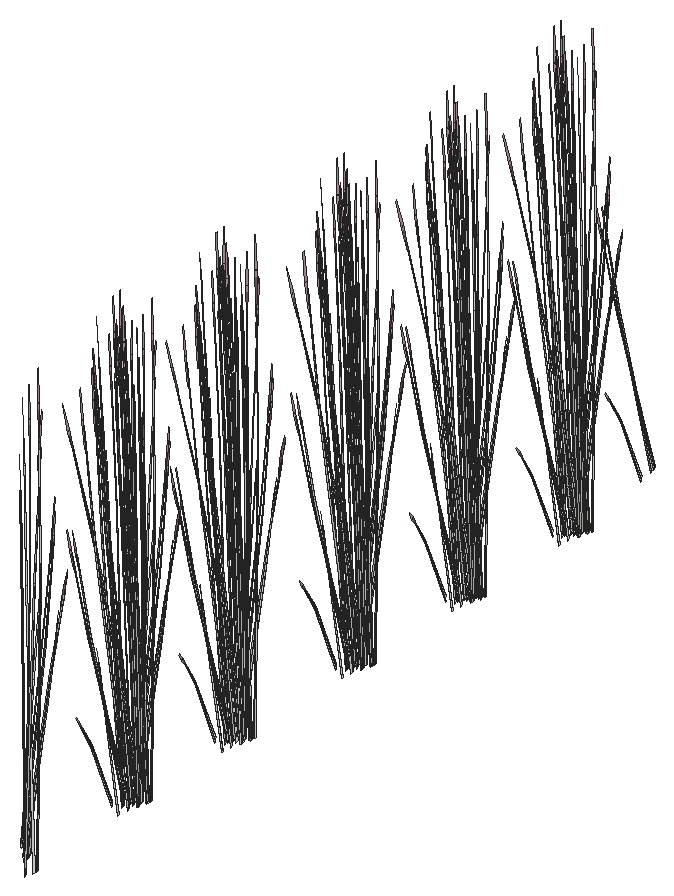
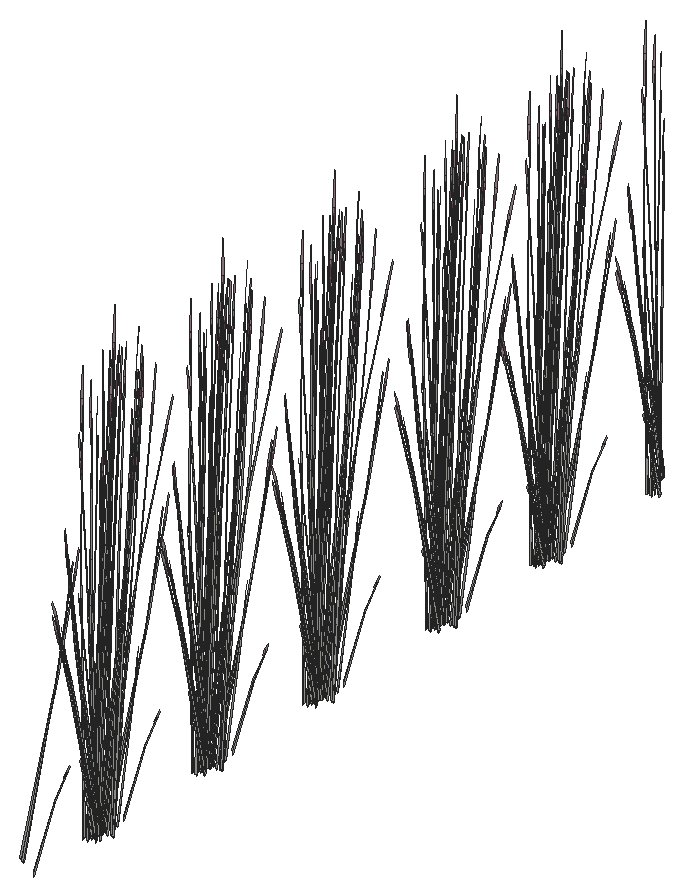
# SketchUp Ruby script. Lengths in inches.
U = 1.inch
M = Sketchup.active_model
def pt(a) = Geom::Point3d.new(a.map { |v| v * U })
def face(e, loops, mat)
  f = e.add_face(loops[0].map { |a| pt(a) })
  loops[1..].each { |l| e.add_face(l.map { |a| pt(a) }).erase! }
  f.material = f.back_material = mat if mat
  f
end
# faces: each face lists its corners as indices into pts; further lists are holes
def faces(e, pts, list, mat = nil) = list.each { |f| face(e, (f[0].is_a?(Array) ? f : [f]).map { |l| l.map { |i| pts[i] } }, mat) }
# xy, xz, yz: faces in a plane at the given z, y or x. An outline is a flat list of corners, or four numbers for a rectangle; further outlines are holes
def ring(l) = l.size == 4 ? [[l[0], l[1]], [l[2], l[1]], [l[2], l[3]], [l[0], l[3]]] : l.each_slice(2).to_a
def flat(e, list, mat, &to3) = list.each { |f| face(e, (f[0].is_a?(Array) ? f : [f]).map { |l| ring(l).map { |u, v| to3.(u, v) } }, mat) }
def xy(e, z, list, mat = nil) = flat(e, list, mat) { |x, y| [x, y, z] }
def xz(e, y, list, mat = nil) = flat(e, list, mat) { |x, z| [x, y, z] }
def yz(e, x, list, mat = nil) = flat(e, list, mat) { |y, z| [x, y, z] }
def lines(e, pts, list) = list.each { |a, b| e.add_line(pt(pts[a]), pt(pts[b])) }
# prism: a flat outline (further loops are holes) pulled along v
def prism(e, loops, v, mat = nil)
  f = face(e, loops, mat); d = Geom::Vector3d.new(v.map { |x| x * U })
  f.pushpull(f.normal.samedirection?(d) ? d.length : -d.length)
end
def box(e, o, s, mat = nil) = prism(e, [[o, [o[0] + s[0], o[1], o[2]], [o[0] + s[0], o[1] + s[1], o[2]], [o[0], o[1] + s[1], o[2]]]], [0, 0, s[2]], mat)
def at(x, y, z, deg = 0) = Geom::Transformation.translation(pt([x, y, z])) * Geom::Transformation.rotation(ORIGIN, Z_AXIS, deg.degrees)
def axes(o, x, y, z) = Geom::Transformation.new([*x, 0, *y, 0, *z, 0, *pt(o).to_a, 1])
def part(name) = M.definitions.add(name)
# library, detail: a bought-in or finely detailed component or shape, given as its bounding box
def library(name, o, s) = part(name).tap { |d| box(d.entities, o, s) }
def detail(e, o, s) = box(e.add_group.entities, o, s)
def put(e, d, t, mat = nil) = e.add_instance(d, t).tap { |i| i.material = mat if mat }
def group(e, t, mat = nil) = e.add_group.tap { |g| g.transformation = t; g.material = mat if mat }.entities
root = M.entities
M.materials.add("LightPink_Translucent").color = [144, 107, 117]
M.materials["LightPink_Translucent"].alpha = 0.75
c1 = part("blade")
p = [[2.15,0.21,22],[0,0.17,0],[0.09,0.45,0],[2.18,0.31,22],[2.29,0.31,22],[0.38,0.45,0],
  [2.48,0.24,33],[2.49,0.24,33],[2.48,0.22,33]]
faces(c1.entities,p,[[0,1,2,3],[4,5,2,3],[6,3,4,7],[8,0,3,6]])
c2 = part("seeds")
p = [[0.3,-0.1,1.38],[-0.01,-0.03,1.59],[-0.01,-0.03,0.03],[0.14,-0.07,-0.07],[0.29,-0.03,3],[0.15,0.01,3.11]]
faces(c2.entities,p,[[0,1,2,3],[1,0,4,5]],"LightPink_Translucent")
c3 = part("blade with seeds")
put(c3.entities,c1,at(0,0,0))
put(c3.entities,c2,axes([2.4,0.25,30.99],[1.5799,-0.05474,1.17369],[-0.12525,1.92788,0.29478],[-0.07173,-0.02425,1.56792]))
put(root,c3,axes([402.46,581.55,2.67],[0.04113,0.53214,-0.29095],[-0.42835,0.03218,-0.50002],[-0.07543,0.07088,1.59708]))
put(root,c3,axes([402.2,581.96,2.06],[-0.23773,0.35053,-0.62353],[-0.29532,-0.31785,-0.16365],[-0.09526,0.08744,1.37633]))
put(root,c3,axes([402.59,582.91,2.02],[-0.33032,0.23318,-0.49651],[-0.19744,-0.41812,0],[-0.07523,0.05311,1.57504]))
put(root,c3,axes([402.89,582.84,2.375],[0.22066,0.46731,0],[-0.36918,0.26061,-0.51607],[-0.08408,0.05936,1.63711]))
put(root,c3,axes([402.7,580.99,2.84],[-0.00964,-0.43909,1.41272],[0.43635,0.11382,0.59816],[-0.1032,0.24027,1.3335]))
put(root,c3,axes([400.98,582.69,4.53],[-0.23881,0.24554,-0.35414],[-0.22606,-0.28036,0.4572],[-0.0344,0.14245,0.87481]))
put(root,c3,axes([401.13,583.64,2.77],[-0.00913,-0.2773,1.1486],[0.22824,0.19778,0.84392],[-0.04489,0.13217,0.25299]))
put(root,c3,axes([401.21,582.57,5],[0.25266,0.31335,-0.5672],[-0.2669,0.27442,-0.43934],[-0.03844,0.15921,1.08528]))
put(root,c3,axes([400.9375,583.04,2.82],[0.32063,-0.08258,0.06507],[0.07371,0.33271,-0.86304],[-0.02033,0.16842,0.7736]))
put(root,c3,axes([401.13,582.43,5.34],[-0.00918,0.43138,-0.7886],[-0.38672,-0.02897,0.09517],[-0.04081,0.18275,1.11556]))
put(root,c3,axes([401.5,582.125,3.875],[-0.00864,-0.17899,1.71376],[0.37441,0.11874,0.13857],[-0.02316,0.25508,0.73262]))
put(root,c3,axes([401.01,583.04,3.36],[0.00775,-0.24075,1.54345],[0.34877,0.12716,0.21329],[-0.03022,0.25658,0.72882]))
put(root,c3,axes([402.27,598.67,4.98],[-0.16845,-0.3792,-0.71045],[0.34676,-0.21133,0.08574],[-0.03939,-0.18322,1.00501]))
put(root,c3,axes([402.14,598.59,4.68],[-0.34695,-0.11691,-0.51099],[0.11892,-0.40083,-0.3958],[-0.03181,-0.16138,0.97773]))
put(root,c3,axes([401.0625,597.91,2.77],[0.18411,0.16231,1.1486],[-0.26813,0.09757,0.84392],[-0.05737,-0.12474,0.25299]))
put(root,c3,axes([401.49,600.09,2.1],[-0.14494,-0.47823,-0.69835],[0.41752,-0.17223,-0.18329],[-0.01602,-0.16194,1.54149]))
put(root,c3,axes([401.92,598.15,2.13],[-0.2439,0.26754,-0.03893],[-0.22348,-0.29302,-0.17649],[-0.01573,-0.08303,0.58215]))
put(root,c3,axes([402.23,601.32,3.33],[0.305,0.18805,1.51261],[-0.29879,0.40513,0.59816],[-0.13384,-0.24012,1.26806]))
put(root,c3,axes([400.63,600.02,2.02],[0,-0.46636,-0.49651],[0.39487,0,0],[0,-0.10622,1.57504]))
put(root,c3,axes([400.8,600.04,2.03],[0.24637,-0.29097,-0.30978],[0.24637,0.29097,0.30978],[0,-0.09372,1.38974]))
put(root,c3,axes([401.67,600.5625,2.67],[-0.39748,-0.22252,-0.29095],[0.19139,-0.46966,-0.50002],[-0.01249,-0.11531,1.59708]))
put(root,c3,axes([400.875,600.24,2.33],[-0.32829,0.39208,0.30756],[-0.32849,-0.38796,-0.36492],[-0.01146,-0.11134,1.64885]))
put(root,c3,axes([401.77,601.06,2.4375],[0.09355,-0.55261,-0.23429],[0.44354,0.09633,0.51271],[-0.0775,-0.07631,1.5644]))
put(root,c3,axes([400.8,600.46,2.48],[0,0.46636,0.49651],[-0.39487,0,0],[0,-0.10622,1.57504]))
put(root,c3,axes([401.73,600.83,2.21],[-0.21202,-0.39143,-0.44739],[0.32115,-0.27564,0.21531],[-0.06861,-0.04843,1.43643]))
put(root,c3,axes([401.7,600.69,2.72],[-0.17124,0.42022,0.44739],[-0.35581,-0.20224,-0.21531],[0,-0.09687,1.43643]))
put(root,c3,axes([402.44,600.74,2.3],[-0.32829,-0.4014,-0.06131],[0.32849,-0.40164,0],[-0.01146,-0.01402,1.75571]))
put(root,c3,axes([401.82,600.79,2.36],[0.44609,0.09826,0.45755],[-0.09078,0.55493,0.17955],[-0.06519,-0.05359,1.58856]))
put(root,c3,axes([401.58,601.68,2.47],[0.37926,-0.12378,0.17642],[0.09365,0.46065,0.35086],[-0.03382,-0.06712,1.60407]))
put(root,c3,axes([401.93,601.1875,2.62],[-0.06809,0.4162,0.1448],[-0.33266,-0.07225,-0.41347],[-0.06054,-0.04274,1.26744]))
put(root,c3,axes([402.71,601.7,2.47],[0.10196,-0.46348,0.17642],[0.3731,0.13116,0.35086],[-0.06445,0.00226,1.60407]))
put(root,c3,axes([402.07,601.75,2.2],[-0.35581,-0.20937,0],[0.17124,-0.43505,0],[0,0,1.62707]))
put(root,c3,axes([402.36,601.19,2.46],[-0.34464,-0.37536,-0.25192],[0.29,-0.42149,0.5513],[-0.0928,0.04391,1.68216]))
put(root,c3,axes([401.45,601.91,2.48],[0.33032,0.23318,0.49651],[-0.19744,0.41812,0],[-0.07523,-0.05311,1.57504]))
put(root,c3,axes([402.53,600.88,2.72],[0.38326,-0.02879,0.44739],[0.03466,0.47788,-0.21531],[-0.06861,0.04843,1.43643]))
put(root,c3,axes([402.1875,601.12,2.21],[-0.38326,0.02879,-0.44739],[-0.03466,-0.47788,0.21531],[-0.06861,0.04843,1.43643]))
put(root,c3,axes([402.61,602.22,2.19],[-0.21791,-0.46895,-0.05142],[0.36918,-0.26061,0.51607],[-0.09097,0.04465,1.6363]))
put(root,c3,axes([402.53,601.09,2.62],[0.26075,0.2802,0.1448],[-0.2175,0.31612,-0.41347],[-0.06054,0.04274,1.26744]))
put(root,c3,axes([402.51,602.16,2.03],[-0.32928,-0.11539,-0.30978],[0.08291,-0.40636,0.30978],[-0.06638,0.04686,1.38974]))
put(root,c3,axes([402.46,600.99,2.67],[0.04113,0.53214,-0.29095],[-0.42835,0.03218,-0.50002],[-0.07543,0.07088,1.59708]))
put(root,c3,axes([402.2,601.39,2.06],[-0.23773,0.35053,-0.62353],[-0.29532,-0.31785,-0.16365],[-0.09526,0.08744,1.37633]))
put(root,c3,axes([402.59,602.35,2.02],[-0.33032,0.23318,-0.49651],[-0.19744,-0.41812,0],[-0.07523,0.05311,1.57504]))
put(root,c3,axes([402.89,602.28,2.375],[0.22066,0.46731,0],[-0.36918,0.26061,-0.51607],[-0.08408,0.05936,1.63711]))
put(root,c3,axes([402.7,600.43,2.84],[-0.00964,-0.43909,1.41272],[0.43635,0.11382,0.59816],[-0.1032,0.24027,1.3335]))
put(root,c3,axes([400.98,602.13,4.53],[-0.23881,0.24554,-0.35414],[-0.22606,-0.28036,0.4572],[-0.0344,0.14245,0.87481]))
put(root,c3,axes([401.13,603.08,2.77],[-0.00913,-0.2773,1.1486],[0.22824,0.19778,0.84392],[-0.04489,0.13217,0.25299]))
put(root,c3,axes([401.21,602.01,5],[0.25266,0.31335,-0.5672],[-0.2669,0.27442,-0.43934],[-0.03844,0.15921,1.08528]))
put(root,c3,axes([400.9375,602.48,2.82],[0.32063,-0.08258,0.06507],[0.07371,0.33271,-0.86304],[-0.02033,0.16842,0.7736]))
put(root,c3,axes([401.13,601.87,5.34],[-0.00918,0.43138,-0.7886],[-0.38672,-0.02897,0.09517],[-0.04081,0.18275,1.11556]))
put(root,c3,axes([401.5,601.5625,3.875],[-0.00864,-0.17899,1.71376],[0.37441,0.11874,0.13857],[-0.02316,0.25508,0.73262]))
put(root,c3,axes([401.01,602.48,3.36],[0.00775,-0.24075,1.54345],[0.34877,0.12716,0.21329],[-0.03022,0.25658,0.72882]))
put(root,c3,axes([402.27,616.25,4.98],[-0.16845,-0.3792,-0.71045],[0.34676,-0.21133,0.08574],[-0.03939,-0.18322,1.00501]))
put(root,c3,axes([402.14,616.17,4.68],[-0.34695,-0.11691,-0.51099],[0.11892,-0.40083,-0.3958],[-0.03181,-0.16138,0.97773]))
put(root,c3,axes([401.0625,615.5,2.77],[0.18411,0.16231,1.1486],[-0.26813,0.09757,0.84392],[-0.05737,-0.12474,0.25299]))
put(root,c3,axes([401.49,617.67,2.1],[-0.14494,-0.47823,-0.69835],[0.41752,-0.17223,-0.18329],[-0.01602,-0.16194,1.54149]))
put(root,c3,axes([401.92,615.74,2.13],[-0.2439,0.26754,-0.03893],[-0.22348,-0.29302,-0.17649],[-0.01573,-0.08303,0.58215]))
put(root,c3,axes([402.23,618.91,3.33],[0.305,0.18805,1.51261],[-0.29879,0.40513,0.59816],[-0.13384,-0.24012,1.26806]))
put(root,c3,axes([400.63,617.61,2.02],[0,-0.46636,-0.49651],[0.39487,0,0],[0,-0.10622,1.57504]))
put(root,c3,axes([400.8,617.62,2.03],[0.24637,-0.29097,-0.30978],[0.24637,0.29097,0.30978],[0,-0.09372,1.38974]))
put(root,c3,axes([401.67,618.15,2.67],[-0.39748,-0.22252,-0.29095],[0.19139,-0.46966,-0.50002],[-0.01249,-0.11531,1.59708]))
put(root,c3,axes([400.875,617.82,2.33],[-0.32829,0.39208,0.30756],[-0.32849,-0.38796,-0.36492],[-0.01146,-0.11134,1.64885]))
put(root,c3,axes([401.77,618.64,2.4375],[0.09355,-0.55261,-0.23429],[0.44354,0.09633,0.51271],[-0.0775,-0.07631,1.5644]))
put(root,c3,axes([400.8,618.04,2.48],[0,0.46636,0.49651],[-0.39487,0,0],[0,-0.10622,1.57504]))
put(root,c3,axes([401.73,618.42,2.21],[-0.21202,-0.39143,-0.44739],[0.32115,-0.27564,0.21531],[-0.06861,-0.04843,1.43643]))
put(root,c3,axes([401.7,618.28,2.72],[-0.17124,0.42022,0.44739],[-0.35581,-0.20224,-0.21531],[0,-0.09687,1.43643]))
put(root,c3,axes([402.44,618.33,2.3],[-0.32829,-0.4014,-0.06131],[0.32849,-0.40164,0],[-0.01146,-0.01402,1.75571]))
put(root,c3,axes([401.82,618.375,2.36],[0.44609,0.09826,0.45755],[-0.09078,0.55493,0.17955],[-0.06519,-0.05359,1.58856]))
put(root,c3,axes([401.58,619.26,2.47],[0.37926,-0.12378,0.17642],[0.09365,0.46065,0.35086],[-0.03382,-0.06712,1.60407]))
put(root,c3,axes([401.93,618.77,2.62],[-0.06809,0.4162,0.1448],[-0.33266,-0.07225,-0.41347],[-0.06054,-0.04274,1.26744]))
put(root,c3,axes([402.71,619.29,2.47],[0.10196,-0.46348,0.17642],[0.3731,0.13116,0.35086],[-0.06445,0.00226,1.60407]))
put(root,c3,axes([402.07,619.34,2.2],[-0.35581,-0.20937,0],[0.17124,-0.43505,0],[0,0,1.62707]))
put(root,c3,axes([402.36,618.78,2.46],[-0.34464,-0.37536,-0.25192],[0.29,-0.42149,0.5513],[-0.0928,0.04391,1.68216]))
put(root,c3,axes([401.45,619.5,2.48],[0.33032,0.23318,0.49651],[-0.19744,0.41812,0],[-0.07523,-0.05311,1.57504]))
put(root,c3,axes([402.53,618.47,2.72],[0.38326,-0.02879,0.44739],[0.03466,0.47788,-0.21531],[-0.06861,0.04843,1.43643]))
put(root,c3,axes([402.1875,618.7,2.21],[-0.38326,0.02879,-0.44739],[-0.03466,-0.47788,0.21531],[-0.06861,0.04843,1.43643]))
put(root,c3,axes([402.61,619.81,2.19],[-0.21791,-0.46895,-0.05142],[0.36918,-0.26061,0.51607],[-0.09097,0.04465,1.6363]))
put(root,c3,axes([402.53,618.67,2.62],[0.26075,0.2802,0.1448],[-0.2175,0.31612,-0.41347],[-0.06054,0.04274,1.26744]))
put(root,c3,axes([402.51,619.75,2.03],[-0.32928,-0.11539,-0.30978],[0.08291,-0.40636,0.30978],[-0.06638,0.04686,1.38974]))
put(root,c3,axes([402.46,618.57,2.67],[0.04113,0.53214,-0.29095],[-0.42835,0.03218,-0.50002],[-0.07543,0.07088,1.59708]))
put(root,c3,axes([402.2,618.97,2.06],[-0.23773,0.35053,-0.62353],[-0.29532,-0.31785,-0.16365],[-0.09526,0.08744,1.37633]))
put(root,c3,axes([402.59,619.93,2.02],[-0.33032,0.23318,-0.49651],[-0.19744,-0.41812,0],[-0.07523,0.05311,1.57504]))
put(root,c3,axes([402.89,619.86,2.375],[0.22066,0.46731,0],[-0.36918,0.26061,-0.51607],[-0.08408,0.05936,1.63711]))
put(root,c3,axes([402.7,618.01,2.84],[-0.00964,-0.43909,1.41272],[0.43635,0.11382,0.59816],[-0.1032,0.24027,1.3335]))
put(root,c3,axes([400.98,619.71,4.53],[-0.23881,0.24554,-0.35414],[-0.22606,-0.28036,0.4572],[-0.0344,0.14245,0.87481]))
put(root,c3,axes([401.13,620.66,2.77],[-0.00913,-0.2773,1.1486],[0.22824,0.19778,0.84392],[-0.04489,0.13217,0.25299]))
put(root,c3,axes([401.21,619.59,5],[0.25266,0.31335,-0.5672],[-0.2669,0.27442,-0.43934],[-0.03844,0.15921,1.08528]))
put(root,c3,axes([400.9375,620.06,2.82],[0.32063,-0.08258,0.06507],[0.07371,0.33271,-0.86304],[-0.02033,0.16842,0.7736]))
put(root,c3,axes([401.13,619.45,5.34],[-0.00918,0.43138,-0.7886],[-0.38672,-0.02897,0.09517],[-0.04081,0.18275,1.11556]))
put(root,c3,axes([401.5,619.14,3.875],[-0.00864,-0.17899,1.71376],[0.37441,0.11874,0.13857],[-0.02316,0.25508,0.73262]))
put(root,c3,axes([401.01,620.06,3.36],[0.00775,-0.24075,1.54345],[0.34877,0.12716,0.21329],[-0.03022,0.25658,0.72882]))
put(root,c3,axes([402.27,636.79,4.98],[-0.16845,-0.3792,-0.71045],[0.34676,-0.21133,0.08574],[-0.03939,-0.18322,1.00501]))
put(root,c3,axes([402.14,636.71,4.68],[-0.34695,-0.11691,-0.51099],[0.11892,-0.40083,-0.3958],[-0.03181,-0.16138,0.97773]))
put(root,c3,axes([401.0625,636.03,2.77],[0.18411,0.16231,1.1486],[-0.26813,0.09757,0.84392],[-0.05737,-0.12474,0.25299]))
put(root,c3,axes([401.49,638.21,2.1],[-0.14494,-0.47823,-0.69835],[0.41752,-0.17223,-0.18329],[-0.01602,-0.16194,1.54149]))
put(root,c3,axes([401.92,636.27,2.13],[-0.2439,0.26754,-0.03893],[-0.22348,-0.29302,-0.17649],[-0.01573,-0.08303,0.58215]))
put(root,c3,axes([402.23,639.44,3.33],[0.305,0.18805,1.51261],[-0.29879,0.40513,0.59816],[-0.13384,-0.24012,1.26806]))
put(root,c3,axes([400.63,638.14,2.02],[0,-0.46636,-0.49651],[0.39487,0,0],[0,-0.10622,1.57504]))
put(root,c3,axes([400.8,638.15,2.03],[0.24637,-0.29097,-0.30978],[0.24637,0.29097,0.30978],[0,-0.09372,1.38974]))
put(root,c3,axes([401.67,638.68,2.67],[-0.39748,-0.22252,-0.29095],[0.19139,-0.46966,-0.50002],[-0.01249,-0.11531,1.59708]))
put(root,c3,axes([400.875,638.36,2.33],[-0.32829,0.39208,0.30756],[-0.32849,-0.38796,-0.36492],[-0.01146,-0.11134,1.64885]))
put(root,c3,axes([401.77,639.18,2.4375],[0.09355,-0.55261,-0.23429],[0.44354,0.09633,0.51271],[-0.0775,-0.07631,1.5644]))
put(root,c3,axes([400.8,638.58,2.48],[0,0.46636,0.49651],[-0.39487,0,0],[0,-0.10622,1.57504]))
put(root,c3,axes([401.73,638.95,2.21],[-0.21202,-0.39143,-0.44739],[0.32115,-0.27564,0.21531],[-0.06861,-0.04843,1.43643]))
put(root,c3,axes([401.7,638.81,2.72],[-0.17124,0.42022,0.44739],[-0.35581,-0.20224,-0.21531],[0,-0.09687,1.43643]))
put(root,c3,axes([402.44,638.86,2.3],[-0.32829,-0.4014,-0.06131],[0.32849,-0.40164,0],[-0.01146,-0.01402,1.75571]))
put(root,c3,axes([401.82,638.91,2.36],[0.44609,0.09826,0.45755],[-0.09078,0.55493,0.17955],[-0.06519,-0.05359,1.58856]))
put(root,c3,axes([401.58,639.8,2.47],[0.37926,-0.12378,0.17642],[0.09365,0.46065,0.35086],[-0.03382,-0.06712,1.60407]))
put(root,c3,axes([401.93,639.31,2.62],[-0.06809,0.4162,0.1448],[-0.33266,-0.07225,-0.41347],[-0.06054,-0.04274,1.26744]))
put(root,c3,axes([402.71,639.82,2.47],[0.10196,-0.46348,0.17642],[0.3731,0.13116,0.35086],[-0.06445,0.00226,1.60407]))
put(root,c3,axes([402.07,639.87,2.2],[-0.35581,-0.20937,0],[0.17124,-0.43505,0],[0,0,1.62707]))
put(root,c3,axes([402.36,639.3125,2.46],[-0.34464,-0.37536,-0.25192],[0.29,-0.42149,0.5513],[-0.0928,0.04391,1.68216]))
put(root,c3,axes([401.45,640.03,2.48],[0.33032,0.23318,0.49651],[-0.19744,0.41812,0],[-0.07523,-0.05311,1.57504]))
put(root,c3,axes([402.53,639,2.72],[0.38326,-0.02879,0.44739],[0.03466,0.47788,-0.21531],[-0.06861,0.04843,1.43643]))
put(root,c3,axes([402.1875,639.23,2.21],[-0.38326,0.02879,-0.44739],[-0.03466,-0.47788,0.21531],[-0.06861,0.04843,1.43643]))
put(root,c3,axes([402.61,640.34,2.19],[-0.21791,-0.46895,-0.05142],[0.36918,-0.26061,0.51607],[-0.09097,0.04465,1.6363]))
put(root,c3,axes([402.53,639.21,2.62],[0.26075,0.2802,0.1448],[-0.2175,0.31612,-0.41347],[-0.06054,0.04274,1.26744]))
put(root,c3,axes([402.51,640.28,2.03],[-0.32928,-0.11539,-0.30978],[0.08291,-0.40636,0.30978],[-0.06638,0.04686,1.38974]))
put(root,c3,axes([402.46,639.1,2.67],[0.04113,0.53214,-0.29095],[-0.42835,0.03218,-0.50002],[-0.07543,0.07088,1.59708]))
put(root,c3,axes([402.2,639.51,2.06],[-0.23773,0.35053,-0.62353],[-0.29532,-0.31785,-0.16365],[-0.09526,0.08744,1.37633]))
put(root,c3,axes([402.59,640.47,2.02],[-0.33032,0.23318,-0.49651],[-0.19744,-0.41812,0],[-0.07523,0.05311,1.57504]))
put(root,c3,axes([402.89,640.39,2.375],[0.22066,0.46731,0],[-0.36918,0.26061,-0.51607],[-0.08408,0.05936,1.63711]))
put(root,c3,axes([402.7,638.54,2.84],[-0.00964,-0.43909,1.41272],[0.43635,0.11382,0.59816],[-0.1032,0.24027,1.3335]))
put(root,c3,axes([400.98,640.24,4.53],[-0.23881,0.24554,-0.35414],[-0.22606,-0.28036,0.4572],[-0.0344,0.14245,0.87481]))
put(root,c3,axes([401.13,641.2,2.77],[-0.00913,-0.2773,1.1486],[0.22824,0.19778,0.84392],[-0.04489,0.13217,0.25299]))
put(root,c3,axes([401.21,640.13,5],[0.25266,0.31335,-0.5672],[-0.2669,0.27442,-0.43934],[-0.03844,0.15921,1.08528]))
put(root,c3,axes([400.9375,640.6,2.82],[0.32063,-0.08258,0.06507],[0.07371,0.33271,-0.86304],[-0.02033,0.16842,0.7736]))
put(root,c3,axes([401.13,639.99,5.34],[-0.00918,0.43138,-0.7886],[-0.38672,-0.02897,0.09517],[-0.04081,0.18275,1.11556]))
put(root,c3,axes([401.5,639.68,3.875],[-0.00864,-0.17899,1.71376],[0.37441,0.11874,0.13857],[-0.02316,0.25508,0.73262]))
put(root,c3,axes([401.01,640.59,3.36],[0.00775,-0.24075,1.54345],[0.34877,0.12716,0.21329],[-0.03022,0.25658,0.72882]))
put(root,c3,axes([402.27,655.46,4.98],[-0.16845,-0.3792,-0.71045],[0.34676,-0.21133,0.08574],[-0.03939,-0.18322,1.00501]))
put(root,c3,axes([402.14,655.38,4.68],[-0.34695,-0.11691,-0.51099],[0.11892,-0.40083,-0.3958],[-0.03181,-0.16138,0.97773]))
put(root,c3,axes([401.0625,654.71,2.77],[0.18411,0.16231,1.1486],[-0.26813,0.09757,0.84392],[-0.05737,-0.12474,0.25299]))
put(root,c3,axes([401.49,656.88,2.1],[-0.14494,-0.47823,-0.69835],[0.41752,-0.17223,-0.18329],[-0.01602,-0.16194,1.54149]))
put(root,c3,axes([401.92,654.95,2.13],[-0.2439,0.26754,-0.03893],[-0.22348,-0.29302,-0.17649],[-0.01573,-0.08303,0.58215]))
put(root,c3,axes([402.23,658.12,3.33],[0.305,0.18805,1.51261],[-0.29879,0.40513,0.59816],[-0.13384,-0.24012,1.26806]))
put(root,c3,axes([400.63,656.82,2.02],[0,-0.46636,-0.49651],[0.39487,0,0],[0,-0.10622,1.57504]))
put(root,c3,axes([400.8,656.83,2.03],[0.24637,-0.29097,-0.30978],[0.24637,0.29097,0.30978],[0,-0.09372,1.38974]))
put(root,c3,axes([401.67,657.36,2.67],[-0.39748,-0.22252,-0.29095],[0.19139,-0.46966,-0.50002],[-0.01249,-0.11531,1.59708]))
put(root,c3,axes([400.875,657.03,2.33],[-0.32829,0.39208,0.30756],[-0.32849,-0.38796,-0.36492],[-0.01146,-0.11134,1.64885]))
put(root,c3,axes([401.77,657.85,2.4375],[0.09355,-0.55261,-0.23429],[0.44354,0.09633,0.51271],[-0.0775,-0.07631,1.5644]))
put(root,c3,axes([400.8,657.25,2.48],[0,0.46636,0.49651],[-0.39487,0,0],[0,-0.10622,1.57504]))
put(root,c3,axes([401.73,657.625,2.21],[-0.21202,-0.39143,-0.44739],[0.32115,-0.27564,0.21531],[-0.06861,-0.04843,1.43643]))
put(root,c3,axes([401.7,657.48,2.72],[-0.17124,0.42022,0.44739],[-0.35581,-0.20224,-0.21531],[0,-0.09687,1.43643]))
put(root,c3,axes([402.44,657.54,2.3],[-0.32829,-0.4014,-0.06131],[0.32849,-0.40164,0],[-0.01146,-0.01402,1.75571]))
put(root,c3,axes([401.82,657.58,2.36],[0.44609,0.09826,0.45755],[-0.09078,0.55493,0.17955],[-0.06519,-0.05359,1.58856]))
put(root,c3,axes([401.58,658.47,2.47],[0.37926,-0.12378,0.17642],[0.09365,0.46065,0.35086],[-0.03382,-0.06712,1.60407]))
put(root,c3,axes([401.93,657.98,2.62],[-0.06809,0.4162,0.1448],[-0.33266,-0.07225,-0.41347],[-0.06054,-0.04274,1.26744]))
put(root,c3,axes([402.71,658.5,2.47],[0.10196,-0.46348,0.17642],[0.3731,0.13116,0.35086],[-0.06445,0.00226,1.60407]))
put(root,c3,axes([402.07,658.54,2.2],[-0.35581,-0.20937,0],[0.17124,-0.43505,0],[0,0,1.62707]))
put(root,c3,axes([402.36,657.99,2.46],[-0.34464,-0.37536,-0.25192],[0.29,-0.42149,0.5513],[-0.0928,0.04391,1.68216]))
put(root,c3,axes([401.45,658.71,2.48],[0.33032,0.23318,0.49651],[-0.19744,0.41812,0],[-0.07523,-0.05311,1.57504]))
put(root,c3,axes([402.53,657.68,2.72],[0.38326,-0.02879,0.44739],[0.03466,0.47788,-0.21531],[-0.06861,0.04843,1.43643]))
put(root,c3,axes([402.1875,657.91,2.21],[-0.38326,0.02879,-0.44739],[-0.03466,-0.47788,0.21531],[-0.06861,0.04843,1.43643]))
put(root,c3,axes([402.61,659.02,2.19],[-0.21791,-0.46895,-0.05142],[0.36918,-0.26061,0.51607],[-0.09097,0.04465,1.6363]))
put(root,c3,axes([402.53,657.88,2.62],[0.26075,0.2802,0.1448],[-0.2175,0.31612,-0.41347],[-0.06054,0.04274,1.26744]))
put(root,c3,axes([402.51,658.96,2.03],[-0.32928,-0.11539,-0.30978],[0.08291,-0.40636,0.30978],[-0.06638,0.04686,1.38974]))
put(root,c3,axes([402.46,657.78,2.67],[0.04113,0.53214,-0.29095],[-0.42835,0.03218,-0.50002],[-0.07543,0.07088,1.59708]))
put(root,c3,axes([402.2,658.18,2.06],[-0.23773,0.35053,-0.62353],[-0.29532,-0.31785,-0.16365],[-0.09526,0.08744,1.37633]))
put(root,c3,axes([402.59,659.14,2.02],[-0.33032,0.23318,-0.49651],[-0.19744,-0.41812,0],[-0.07523,0.05311,1.57504]))
put(root,c3,axes([402.89,659.07,2.375],[0.22066,0.46731,0],[-0.36918,0.26061,-0.51607],[-0.08408,0.05936,1.63711]))
put(root,c3,axes([402.7,657.22,2.84],[-0.00964,-0.43909,1.41272],[0.43635,0.11382,0.59816],[-0.1032,0.24027,1.3335]))
put(root,c3,axes([400.98,658.92,4.53],[-0.23881,0.24554,-0.35414],[-0.22606,-0.28036,0.4572],[-0.0344,0.14245,0.87481]))
put(root,c3,axes([401.13,659.87,2.77],[-0.00913,-0.2773,1.1486],[0.22824,0.19778,0.84392],[-0.04489,0.13217,0.25299]))
put(root,c3,axes([401.21,658.8,5],[0.25266,0.31335,-0.5672],[-0.2669,0.27442,-0.43934],[-0.03844,0.15921,1.08528]))
put(root,c3,axes([400.9375,659.27,2.82],[0.32063,-0.08258,0.06507],[0.07371,0.33271,-0.86304],[-0.02033,0.16842,0.7736]))
put(root,c3,axes([401.13,658.66,5.34],[-0.00918,0.43138,-0.7886],[-0.38672,-0.02897,0.09517],[-0.04081,0.18275,1.11556]))
put(root,c3,axes([401.5,658.35,3.875],[-0.00864,-0.17899,1.71376],[0.37441,0.11874,0.13857],[-0.02316,0.25508,0.73262]))
put(root,c3,axes([401.01,659.27,3.36],[0.00775,-0.24075,1.54345],[0.34877,0.12716,0.21329],[-0.03022,0.25658,0.72882]))
put(root,c3,axes([402.27,673.67,4.98],[-0.16845,-0.3792,-0.71045],[0.34676,-0.21133,0.08574],[-0.03939,-0.18322,1.00501]))
put(root,c3,axes([402.14,673.6,4.68],[-0.34695,-0.11691,-0.51099],[0.11892,-0.40083,-0.3958],[-0.03181,-0.16138,0.97773]))
put(root,c3,axes([401.0625,672.92,2.77],[0.18411,0.16231,1.1486],[-0.26813,0.09757,0.84392],[-0.05737,-0.12474,0.25299]))
put(root,c3,axes([401.49,675.1,2.1],[-0.14494,-0.47823,-0.69835],[0.41752,-0.17223,-0.18329],[-0.01602,-0.16194,1.54149]))
put(root,c3,axes([401.92,673.16,2.13],[-0.2439,0.26754,-0.03893],[-0.22348,-0.29302,-0.17649],[-0.01573,-0.08303,0.58215]))
put(root,c3,axes([402.23,676.33,3.33],[0.305,0.18805,1.51261],[-0.29879,0.40513,0.59816],[-0.13384,-0.24012,1.26806]))
put(root,c3,axes([400.63,675.03,2.02],[0,-0.46636,-0.49651],[0.39487,0,0],[0,-0.10622,1.57504]))
put(root,c3,axes([400.8,675.04,2.03],[0.24637,-0.29097,-0.30978],[0.24637,0.29097,0.30978],[0,-0.09372,1.38974]))
put(root,c3,axes([401.67,675.57,2.67],[-0.39748,-0.22252,-0.29095],[0.19139,-0.46966,-0.50002],[-0.01249,-0.11531,1.59708]))
put(root,c3,axes([400.875,675.25,2.33],[-0.32829,0.39208,0.30756],[-0.32849,-0.38796,-0.36492],[-0.01146,-0.11134,1.64885]))
put(root,c3,axes([401.77,676.07,2.4375],[0.09355,-0.55261,-0.23429],[0.44354,0.09633,0.51271],[-0.0775,-0.07631,1.5644]))
put(root,c3,axes([400.8,675.46,2.48],[0,0.46636,0.49651],[-0.39487,0,0],[0,-0.10622,1.57504]))
put(root,c3,axes([401.73,675.84,2.21],[-0.21202,-0.39143,-0.44739],[0.32115,-0.27564,0.21531],[-0.06861,-0.04843,1.43643]))
put(root,c3,axes([401.7,675.7,2.72],[-0.17124,0.42022,0.44739],[-0.35581,-0.20224,-0.21531],[0,-0.09687,1.43643]))
put(root,c3,axes([402.44,675.75,2.3],[-0.32829,-0.4014,-0.06131],[0.32849,-0.40164,0],[-0.01146,-0.01402,1.75571]))
put(root,c3,axes([401.82,675.8,2.36],[0.44609,0.09826,0.45755],[-0.09078,0.55493,0.17955],[-0.06519,-0.05359,1.58856]))
put(root,c3,axes([401.15,676.71,2.03],[-0.08291,-0.40636,-0.30978],[0.32928,-0.11539,0.30978],[-0.06638,-0.04686,1.38974]))
put(root,c3,axes([401.58,676.6875,2.47],[0.37926,-0.12378,0.17642],[0.09365,0.46065,0.35086],[-0.03382,-0.06712,1.60407]))
put(root,c3,axes([401.93,676.2,2.62],[-0.06809,0.4162,0.1448],[-0.33266,-0.07225,-0.41347],[-0.06054,-0.04274,1.26744]))
put(root,c3,axes([402.71,676.71,2.47],[0.10196,-0.46348,0.17642],[0.3731,0.13116,0.35086],[-0.06445,0.00226,1.60407]))
put(root,c3,axes([402.07,676.76,2.2],[-0.35581,-0.20937,0],[0.17124,-0.43505,0],[0,0,1.62707]))
put(root,c3,axes([402.36,676.2,2.46],[-0.34464,-0.37536,-0.25192],[0.29,-0.42149,0.5513],[-0.0928,0.04391,1.68216]))
put(root,c3,axes([401.45,676.92,2.48],[0.33032,0.23318,0.49651],[-0.19744,0.41812,0],[-0.07523,-0.05311,1.57504]))
put(root,c3,axes([402.1875,676.12,2.21],[-0.38326,0.02879,-0.44739],[-0.03466,-0.47788,0.21531],[-0.06861,0.04843,1.43643]))
put(root,c3,axes([402.61,677.23,2.19],[-0.21791,-0.46895,-0.05142],[0.36918,-0.26061,0.51607],[-0.09097,0.04465,1.6363]))
put(root,c3,axes([402.53,676.1,2.62],[0.26075,0.2802,0.1448],[-0.2175,0.31612,-0.41347],[-0.06054,0.04274,1.26744]))
put(root,c3,axes([402.51,677.17,2.03],[-0.32928,-0.11539,-0.30978],[0.08291,-0.40636,0.30978],[-0.06638,0.04686,1.38974]))
put(root,c3,axes([402.46,675.99,2.67],[0.04113,0.53214,-0.29095],[-0.42835,0.03218,-0.50002],[-0.07543,0.07088,1.59708]))
put(root,c3,axes([402.2,676.4,2.06],[-0.23773,0.35053,-0.62353],[-0.29532,-0.31785,-0.16365],[-0.09526,0.08744,1.37633]))
put(root,c3,axes([402.59,677.36,2.02],[-0.33032,0.23318,-0.49651],[-0.19744,-0.41812,0],[-0.07523,0.05311,1.57504]))
put(root,c3,axes([402.89,677.28,2.375],[0.22066,0.46731,0],[-0.36918,0.26061,-0.51607],[-0.08408,0.05936,1.63711]))
put(root,c3,axes([402.7,675.43,2.84],[-0.00964,-0.43909,1.41272],[0.43635,0.11382,0.59816],[-0.1032,0.24027,1.3335]))
put(root,c3,axes([400.98,677.13,4.53],[-0.23881,0.24554,-0.35414],[-0.22606,-0.28036,0.4572],[-0.0344,0.14245,0.87481]))
put(root,c3,axes([401.13,678.09,2.77],[-0.00913,-0.2773,1.1486],[0.22824,0.19778,0.84392],[-0.04489,0.13217,0.25299]))
put(root,c3,axes([401.21,677.02,5],[0.25266,0.31335,-0.5672],[-0.2669,0.27442,-0.43934],[-0.03844,0.15921,1.08528]))
put(root,c3,axes([400.9375,677.49,2.82],[0.32063,-0.08258,0.06507],[0.07371,0.33271,-0.86304],[-0.02033,0.16842,0.7736]))
put(root,c3,axes([401.13,676.875,5.34],[-0.00918,0.43138,-0.7886],[-0.38672,-0.02897,0.09517],[-0.04081,0.18275,1.11556]))
put(root,c3,axes([401.5,676.57,3.875],[-0.00864,-0.17899,1.71376],[0.37441,0.11874,0.13857],[-0.02316,0.25508,0.73262]))
put(root,c3,axes([401.01,677.48,3.36],[0.00775,-0.24075,1.54345],[0.34877,0.12716,0.21329],[-0.03022,0.25658,0.72882]))
put(root,c3,axes([402.27,688.75,4.98],[-0.16845,-0.3792,-0.71045],[0.34676,-0.21133,0.08574],[-0.03939,-0.18322,1.00501]))
put(root,c3,axes([402.14,688.67,4.68],[-0.34695,-0.11691,-0.51099],[0.11892,-0.40083,-0.3958],[-0.03181,-0.16138,0.97773]))
put(root,c3,axes([401.0625,688,2.77],[0.18411,0.16231,1.1486],[-0.26813,0.09757,0.84392],[-0.05737,-0.12474,0.25299]))
